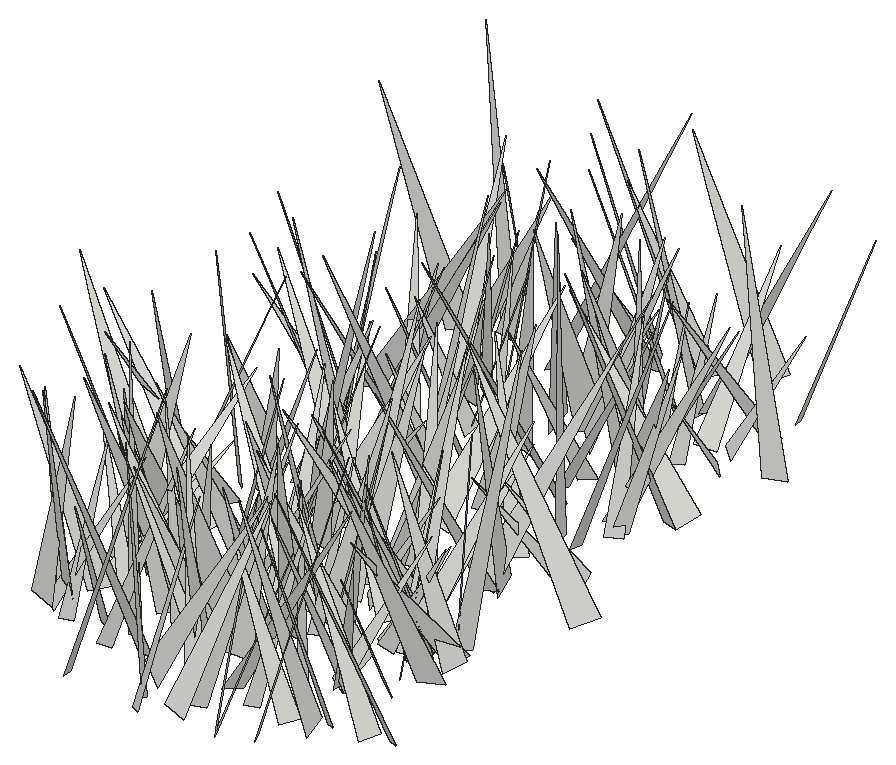
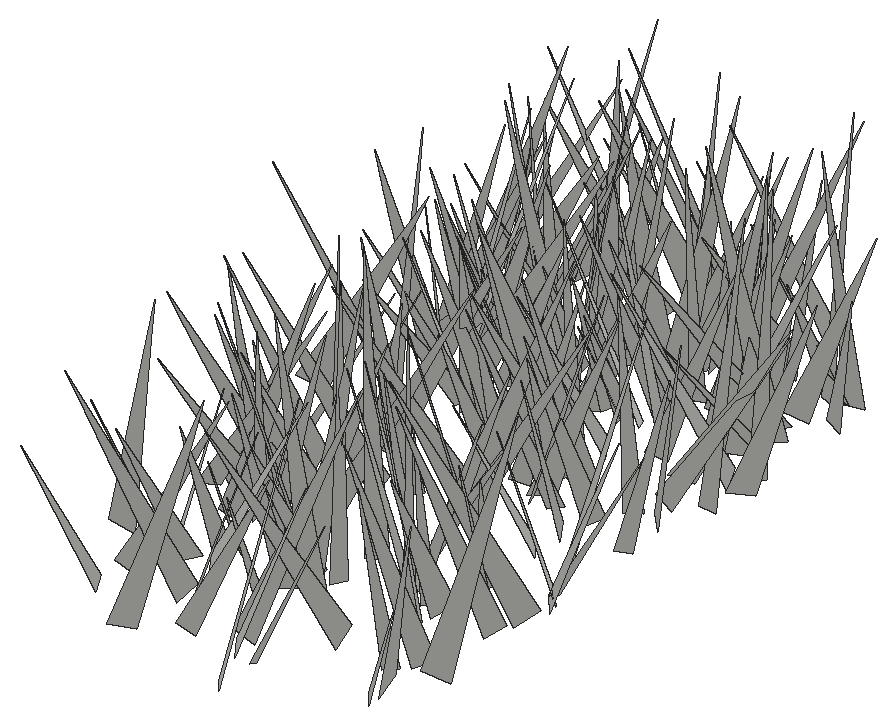
# SketchUp Ruby script. Lengths in inches.
U = 1.inch
M = Sketchup.active_model
def pt(a) = Geom::Point3d.new(a.map { |v| v * U })
def face(e, loops, mat)
  f = e.add_face(loops[0].map { |a| pt(a) })
  loops[1..].each { |l| e.add_face(l.map { |a| pt(a) }).erase! }
  f.material = f.back_material = mat if mat
  f
end
# faces: each face lists its corners as indices into pts; further lists are holes
def faces(e, pts, list, mat = nil) = list.each { |f| face(e, (f[0].is_a?(Array) ? f : [f]).map { |l| l.map { |i| pts[i] } }, mat) }
# xy, xz, yz: faces in a plane at the given z, y or x. An outline is a flat list of corners, or four numbers for a rectangle; further outlines are holes
def ring(l) = l.size == 4 ? [[l[0], l[1]], [l[2], l[1]], [l[2], l[3]], [l[0], l[3]]] : l.each_slice(2).to_a
def flat(e, list, mat, &to3) = list.each { |f| face(e, (f[0].is_a?(Array) ? f : [f]).map { |l| ring(l).map { |u, v| to3.(u, v) } }, mat) }
def xy(e, z, list, mat = nil) = flat(e, list, mat) { |x, y| [x, y, z] }
def xz(e, y, list, mat = nil) = flat(e, list, mat) { |x, z| [x, y, z] }
def yz(e, x, list, mat = nil) = flat(e, list, mat) { |y, z| [x, y, z] }
def lines(e, pts, list) = list.each { |a, b| e.add_line(pt(pts[a]), pt(pts[b])) }
# prism: a flat outline (further loops are holes) pulled along v
def prism(e, loops, v, mat = nil)
  f = face(e, loops, mat); d = Geom::Vector3d.new(v.map { |x| x * U })
  f.pushpull(f.normal.samedirection?(d) ? d.length : -d.length)
end
def box(e, o, s, mat = nil) = prism(e, [[o, [o[0] + s[0], o[1], o[2]], [o[0] + s[0], o[1] + s[1], o[2]], [o[0], o[1] + s[1], o[2]]]], [0, 0, s[2]], mat)
def at(x, y, z, deg = 0) = Geom::Transformation.translation(pt([x, y, z])) * Geom::Transformation.rotation(ORIGIN, Z_AXIS, deg.degrees)
def axes(o, x, y, z) = Geom::Transformation.new([*x, 0, *y, 0, *z, 0, *pt(o).to_a, 1])
def part(name) = M.definitions.add(name)
# library, detail: a bought-in or finely detailed component or shape, given as its bounding box
def library(name, o, s) = part(name).tap { |d| box(d.entities, o, s) }
def detail(e, o, s) = box(e.add_group.entities, o, s)
def put(e, d, t, mat = nil) = e.add_instance(d, t).tap { |i| i.material = mat if mat }
def group(e, t, mat = nil) = e.add_group.tap { |g| g.transformation = t; g.material = mat if mat }.entities
root = M.entities
c1 = part("fur_instance\#9")
p = [[0.8125,0,1.79],[0.67,-0.02,1.48],[0,-0.11,0],[0,0.11,0]]
faces(c1.entities,p,[[0,1,2,3]])
put(root,c1,axes([454.45,326.67,-21.66],[-5.80896,4.38047,0.69826],[4.41604,5.60261,1.59041],[-0.41794,-1.68592,7.09952]))
put(root,c1,axes([454.91,341.82,-21.66],[-4.61833,-3.74237,0.73758],[-3.79853,4.40694,-1.4242],[-0.34716,1.56584,5.77113]))
put(root,c1,axes([456,353.72,-21.66],[-7.80069,-0.47128,0.71432],[-0.70737,7.23754,-2.94972],[0.48165,2.99651,7.23686]))
put(root,c1,axes([454.72,351.37,-21.66],[1.74253,-7.39949,2.19817],[-7.33714,-2.28781,-1.88496],[-2.39807,1.62304,7.36449]))
put(root,c1,axes([455.25,340.96,-21.66],[-4.70731,-0.314,0.0439],[-0.28456,4.4722,1.47573],[0.13983,-1.46975,4.48103]))
put(root,c1,axes([455.15,318.15,-21.66],[0.45308,4.94253,1.25959],[4.74966,-0.86975,1.70432],[-1.859,-1.01755,4.66145]))
put(root,c1,axes([457.82,327.3125,-21.66],[-5.05806,4.73106,0.08976],[4.36112,4.60989,2.7757],[-1.83619,-2.08349,6.34527]))
put(root,c1,axes([456.97,329.83,-21.66],[-0.73144,-5.99959,0.26703],[-5.39662,0.53861,-2.681],[-2.63493,0.56233,5.41685]))
put(root,c1,axes([455.95,355.36,-21.66],[-3.1769,-1.92196,0.83625],[-2.09296,2.82701,-1.45378],[-0.11299,1.67333,3.4166]))
put(root,c1,axes([456.02,331.62,-21.66],[-4.69579,-3.74143,2.09942],[-4.25802,4.44495,-1.60248],[0.52452,2.58851,5.78625]))
put(root,c1,axes([457.25,318.62,-21.66],[-3.27496,5.22829,1.96451],[5.47571,2.5569,2.32348],[-1.10043,-2.83671,5.71505]))
put(root,c1,axes([455.21,341.04,-21.66],[4.3588,4.87451,1.02077],[4.50794,-4.43827,1.9448],[-2.11691,0.58556,6.24322]))
put(root,c1,axes([455.375,335.16,-21.66],[3.46395,-3.11936,0.86631],[-2.7787,-3.51575,-1.54862],[-1.66124,-0.62369,4.39672]))
put(root,c1,axes([454.77,328.99,-21.66],[-2.27672,-7.40144,1.23154],[-7.29478,2.48469,1.44709],[1.75622,0.72557,7.60728]))
put(root,c1,axes([456.03,339.17,-21.66],[-4.76858,-5.56642,0.65425],[-5.40433,4.79429,1.40014],[1.48534,-0.42682,7.19472]))
put(root,c1,axes([459.25,321.66,-21.66],[-5.59942,-5.49473,0.70955],[-5.42162,5.22657,-2.3104],[-1.14084,2.13071,7.49717]))
put(root,c1,axes([458.1,321.33,-21.66],[-3.16034,-1.96863,0.75138],[-2.10046,2.8354,-1.40585],[-0.16774,1.5852,3.44773]))
put(root,c1,axes([454.72,324.94,-21.66],[-1.50636,-7.45489,0.25307],[-6.77182,1.47502,3.14252],[3.12761,-0.39686,6.92598]))
put(root,c1,axes([458.41,342.57,-21.66],[-4.8792,2.06982,0.10093],[1.96371,4.70056,-1.46614],[0.66196,1.31208,5.09325]))
put(root,c1,axes([455.55,315.87,-21.66],[-0.42435,-6.57592,2.54627],[-6.78158,1.0798,1.65847],[1.93298,2.34469,6.37748]))
put(root,c1,axes([455.8,345.44,-21.66],[1.53162,3.70831,1.75315],[4.01532,-0.97314,-1.44953],[0.83802,-2.1148,3.74116]))
put(root,c1,axes([457.88,314.98,-21.66],[-4.70225,1.57903,0.9136],[0.9953,4.33742,-2.37389],[1.52885,2.03289,4.35536]))
put(root,c1,axes([459.29,318.37,-21.66],[-1.35626,4.67986,0.4324],[4.48876,1.15652,1.56235],[-1.3925,-0.82998,4.61514]))
put(root,c1,axes([455.82,325.75,-21.66],[6.85876,3.23862,0.41321],[3.02392,-6.66397,2.03701],[-1.23097,1.67477,7.30628]))
put(root,c1,axes([458.6875,345.74,-21.66],[-5.84983,3.65343,0.11485],[3.32744,5.4123,-2.68634],[1.51292,2.22277,6.35229]))
put(root,c1,axes([457.08,316.24,-21.66],[-3.46246,-6.72611,1.90114],[-6.59046,3.84836,1.61233],[2.32826,0.89059,7.39118]))
put(root,c1,axes([457.16,323.55,-21.66],[4.65411,-4.15615,0.09318],[-4.0063,-4.52139,-1.56511],[-1.10988,-1.10744,6.04026]))
put(root,c1,axes([456.25,322.54,-21.66],[-0.23722,4.19444,0.05409],[3.55446,0.22976,-2.22834],[2.22756,0.08005,3.56147]))
put(root,c1,axes([455.27,345.79,-21.66],[6.30652,-2.10429,0.15189],[-2.07978,-6.12031,1.56194],[0.35446,1.52876,6.46224]))
put(root,c1,axes([454.82,343.72,-21.66],[6.90826,-2.9112,0.5406],[-2.88435,-6.30625,2.89882],[0.66922,2.87186,6.91346]))
put(root,c1,axes([457.01,352.21,-21.66],[1.41484,-4.55258,1.06253],[-4.54528,-1.07998,1.42506],[1.09333,1.40157,4.54939]))
put(root,c1,axes([461.44,318.69,-21.66],[0.20171,6.63601,2.13173],[6.14884,-1.17367,3.07178],[-3.28217,-1.79094,5.8857]))
put(root,c1,axes([456.18,315.875,-21.66],[3.26284,4.45559,0.15103],[4.26787,-3.06768,-1.7017],[1.28856,-1.1217,5.25381]))
put(root,c1,axes([456,350.75,-21.66],[4.35594,-4.3452,0.48537],[-4.22774,-4.01128,2.03138],[1.11472,1.7662,5.80763]))
put(root,c1,axes([459.2,335.46,-21.66],[4.53649,3.63122,1.57008],[3.09166,-4.74451,2.04009],[-2.46831,0.73111,5.44092]))
put(root,c1,axes([456.54,321.33,-21.66],[0.11593,7.32982,3.76994],[7.80213,1.11829,-2.4142],[2.6581,-3.60212,6.9218]))
put(root,c1,axes([460.31,326.29,-21.66],[2.04194,-5.37013,1.21962],[-4.97283,-2.35693,-2.05211],[-2.36574,0.31918,5.36625]))
put(root,c1,axes([457.5,331.64,-21.66],[0.9975,-5.62203,0.93729],[-5.55991,-0.75041,1.41599],[1.25425,1.14473,5.53148]))
put(root,c1,axes([457.11,320.0625,-21.66],[-1.44675,6.62808,0.1342],[5.91861,1.35324,-3.03008],[2.98656,0.529,6.06986]))
put(root,c1,axes([462.35,333.15,-21.66],[-5.71185,4.45959,0.23835],[4.39877,5.55102,1.55146],[-0.77178,-1.36683,7.07857]))
put(root,c1,axes([458.05,324.46,-21.66],[7.18044,-3.7228,0.21814],[-3.29243,-6.55088,-3.42221],[-1.75122,-2.94828,7.32847]))
put(root,c1,axes([460.53,320.83,-21.66],[0.98136,-7.62341,0.77855],[-7.49654,-1.11781,-1.49599],[-1.58884,0.56543,7.53933]))
put(root,c1,axes([462.77,333.13,-21.66],[-7.75285,-2.01113,0.68817],[-2.11722,7.53738,-1.82488],[0.1887,1.94117,7.79879]))
put(root,c1,axes([461.73,315.84,-21.66],[2.76553,6.92914,2.18566],[6.51494,-3.40021,2.53621],[-3.21647,-0.92942,7.01632]))
put(root,c1,axes([459.09,337.72,-21.66],[4.51704,3.2359,0.24642],[3.07452,-4.40221,1.45028],[-1.0388,1.04161,5.3639]))
put(root,c1,axes([458.46,333.63,-21.66],[4.54931,-2.96003,1.24819],[-3.21199,-4.22741,1.68171],[-0.05363,2.09362,5.16041]))
put(root,c1,axes([463.15,340.97,-21.66],[-3.16767,-3.69393,0.44061],[-3.42422,2.66901,-2.24153],[-1.45395,1.76199,4.31912]))
put(root,c1,axes([463.41,314.64,-21.66],[-3.74944,-6.99723,1.04952],[-6.92154,3.38084,-2.18706],[-1.468,1.93125,7.63127]))
put(root,c1,axes([460.03,315.61,-21.66],[-1.799,-4.93024,0.4482],[-4.7112,1.85147,1.45641],[1.52075,-0.09654,5.04207]))
put(root,c1,axes([463.7,337.92,-21.66],[-2.5504,-6.61055,0.06946],[-6.29815,2.40698,-2.17909],[-2.00934,0.84606,6.74207]))
put(root,c1,axes([461.82,343.42,-21.66],[-4.35378,0.44066,1.23045],[0.84047,4.2213,1.46212],[1.0009,-1.62788,4.12453]))
put(root,c1,axes([460.77,331.1,-21.66],[7.1916,2.06862,2.54607],[1.20326,-7.37063,2.58975],[-3.05186,1.96861,7.0208]))
put(root,c1,axes([458.76,347.55,-21.66],[5.69332,3.04756,1.30745],[3.31373,-5.12843,-2.47574],[0.12746,-2.79687,5.96424]))
put(root,c1,axes([459.66,345.77,-21.66],[0.42063,-4.67833,0.35233],[-4.37367,-0.26302,1.72907],[1.69763,0.48155,4.36738]))
put(root,c1,axes([461.125,314.07,-21.66],[-5.44791,2.04028,1.98238],[0.64646,5.0587,-3.42987],[2.77031,2.83181,4.69878]))
put(root,c1,axes([462.67,331.28,-21.66],[-4.26385,3.34064,0.29483],[3.15748,4.15963,-1.468],[1.13011,0.98225,5.21395]))
put(root,c1,axes([463.83,316.89,-21.66],[-6.21207,0.31771,0.7174],[0.09871,5.99609,-1.80072],[0.77837,1.77522,5.95384]))
put(root,c1,axes([462.92,356.15,-21.66],[-3.99864,-1.03805,0.42764],[-0.78188,3.71014,1.695],[0.80565,-1.55139,3.76744]))
put(root,c1,axes([464.61,355.43,-21.66],[-5.23852,-3.39609,0.6769],[-3.443,4.97658,-1.67721],[-0.37061,1.77027,6.01352]))
put(root,c1,axes([461.47,310.59,-21.66],[6.96857,3.90701,1.2479],[3.36407,-6.85211,2.66731],[-2.34628,1.77954,7.53068]))
put(root,c1,axes([464.39,318.08,-21.66],[-6.62778,2.24684,1.33683],[2.5489,6.36376,1.94128],[0.58185,-2.2841,6.72363]))
put(root,c1,axes([460.31,346.55,-21.66],[-2.5118,-6.70095,1.69222],[-6.07027,2.9998,2.86854],[3.30427,0.41708,6.55616]))
put(root,c1,axes([464.28,337.13,-21.66],[-0.7633,-7.78268,1.04828],[-7.63293,0.4877,-1.93706],[-1.84592,1.20152,7.57632]))
put(root,c1,axes([462.84,359.08,-21.66],[-6.10663,-5.12788,1.30944],[-4.81653,6.21333,1.86984],[2.19336,-0.63253,7.75176]))
put(root,c1,axes([462.75,338.36,-21.66],[4.10406,6.33899,0.98584],[6.11766,-4.2195,1.66374],[-1.93105,0.10466,7.36601]))
put(root,c1,axes([461.02,351.08,-21.66],[7.74445,1.42991,0.81828],[1.0012,-7.20795,3.11989],[-1.30836,2.94814,7.231]))
put(root,c1,axes([463.49,343.16,-21.66],[5.66789,4.81372,1.80284],[4.22946,-5.89252,2.43659],[-2.92126,0.80836,7.02566]))
put(root,c1,axes([460.75,325.09,-21.66],[6.83601,2.20523,1.02382],[2.40175,-6.59991,-1.82073],[-0.37792,-2.05437,6.94831]))
put(root,c1,axes([462.76,327.26,-21.66],[5.4592,3.52611,0.65952],[3.05756,-5.20187,2.50265],[-1.87611,1.78282,5.99776]))
put(root,c1,axes([462.05,323.25,-21.66],[6.79493,0.95964,1.40947],[0.56386,-6.72962,1.86359],[-1.60922,1.6941,6.60447]))
put(root,c1,axes([460.98,333.67,-21.66],[0.71966,5.69009,1.64056],[5.43341,0.02279,-2.46251],[2.35511,-1.79132,5.17987]))
put(root,c1,axes([461.04,344.66,-21.66],[5.75664,2.23558,0.62086],[2.31995,-5.52205,-1.62697],[0.03364,-1.74108,5.95732]))
put(root,c1,axes([465.04,354.21,-21.66],[-0.88458,-7.33954,0.10795],[-7.20369,0.84713,-1.43254],[-1.40973,0.27658,7.25253]))
put(root,c1,axes([464.45,338.03,-21.66],[1.33499,-4.14938,1.03511],[-3.92508,-1.61935,-1.42916],[-1.69781,0.48101,4.1179]))
put(root,c1,axes([462.26,320.4,-21.66],[-0.76172,-5.93829,1.58025],[-5.83151,1.20063,1.7008],[1.93753,1.27903,5.74028]))
put(root,c1,axes([466.95,323.11,-21.66],[-5.54363,5.04114,0.10568],[4.92423,5.3789,1.72499],[-1.08457,-1.34553,7.29173]))
put(root,c1,axes([465.28,318.05,-21.66],[1.50286,-5.49819,1.33251],[-5.18917,-1.88889,-1.94134],[-2.25347,0.68284,5.35909]))
put(root,c1,axes([466.13,311.1,-21.66],[-6.09623,-2.24198,1.5344],[-2.70516,5.35755,-2.91953],[0.25098,3.28863,5.80232]))
put(root,c1,axes([464.22,324.01,-21.66],[-4.08665,1.67614,0.95166],[1.15635,3.91687,-1.93308],[1.54207,1.50482,3.97156]))
put(root,c1,axes([463.8,320.8,-21.66],[5.79186,-5.56058,1.06137],[-5.14067,-5.80215,-2.34538],[-2.37068,-1.00358,7.67886]))
put(root,c1,axes([464.09,332.76,-21.66],[4.06405,-3.6671,0.18626],[-3.28339,-3.75381,-2.26428],[-1.64366,-1.56845,4.98369]))
put(root,c1,axes([464.62,324.06,-21.66],[2.09645,3.63188,0.13416],[3.39461,-2.01213,1.42535],[-1.29816,0.60366,3.94386]))
put(root,c1,axes([465.27,323.62,-21.66],[-4.827,3.94667,0.05385],[3.76525,4.62978,-1.80751],[1.18405,1.36675,5.96733]))
put(root,c1,axes([462.75,321.3,-21.66],[4.25693,-2.37845,0.80532],[-2.50825,-3.95225,1.586],[0.11926,1.77474,4.61119]))
put(root,c1,axes([463.29,329.15,-21.66],[0.26156,-6.27199,1.2943],[-6.21893,0.06053,1.55008],[1.52905,1.31908,6.08306]))
put(root,c1,axes([466.35,339.27,-21.66],[1.43264,6.02249,0.66756],[5.77311,-1.565,1.72927],[-1.84042,-0.22107,5.94411]))
put(root,c1,axes([467.85,355.51,-21.66],[-2.55985,4.83206,1.74885],[4.89019,1.69025,2.4878],[-1.579,-2.59892,4.86955]))
put(root,c1,axes([462.39,330.15,-21.66],[3.74419,-3.98525,0.35569],[-3.51637,-3.04515,2.89653],[1.90889,2.20738,4.63803]))
put(root,c1,axes([467.35,313.7,-21.66],[0.02975,6.47261,1.15989],[6.34372,-0.33363,1.69906],[-1.73125,-1.11127,6.2457]))
put(root,c1,axes([465.97,324.68,-21.66],[6.61822,-2.56323,1.80089],[-1.74555,-6.51281,-2.85492],[-2.60123,-2.15113,6.49773]))
put(root,c1,axes([462.99,324.16,-21.66],[5.8637,3.4963,0.04079],[3.31459,-5.53283,-2.23832],[1.11324,-1.94227,6.44958]))
put(root,c1,axes([464.78,346.78,-21.66],[7.73874,0.04549,1.82687],[0.5794,-7.60007,-2.26513],[-1.73315,-2.33761,7.39995]))
put(root,c1,axes([465.82,348.07,-21.66],[6.63906,-4.24471,1.17982],[-3.75911,-6.57064,-2.48644],[-2.29753,-1.51516,7.47745]))
put(root,c1,axes([466.73,331.93,-21.66],[-5.00496,1.9066,1.35129],[1.19771,4.83542,-2.3864],[2.00664,1.8693,4.79477]))
put(root,c1,axes([466.52,309.85,-21.66],[3.68113,4.53912,0.36663],[4.24955,-3.59341,1.82137],[-1.63686,0.87892,5.5531]))
put(root,c1,axes([469.94,340.55,-21.66],[-3.80092,-6.72254,0.0507],[-6.48684,3.65215,-2.05545],[-1.76524,1.05421,7.4441]))
put(root,c1,axes([464.75,343.61,-21.66],[-0.13317,-8.12567,1.45261],[-7.87911,0.55826,2.40046],[2.46092,1.34765,7.76415]))
put(root,c1,axes([469.95,351.98,-21.66],[-6.83624,-2.0461,0.45627],[-2.08301,6.45462,-2.26447],[-0.23611,2.29788,6.76704]))
put(root,c1,axes([466.48,315.76,-21.66],[6.75782,0.35235,2.65885],[1.16075,-6.88187,-2.03823],[-2.41791,-2.31896,6.45275]))
put(root,c1,axes([467.33,350.28,-21.66],[3.33394,1.47543,1.26624],[0.9738,-3.44268,1.44745],[-1.68284,0.93087,3.34618]))
put(root,c1,axes([465.17,348.33,-21.66],[0.9927,-7.18833,2.00129],[-7.23058,-0.4281,2.04891],[1.84279,2.19257,6.96128]))
put(root,c1,axes([467.72,324.23,-21.66],[-6.44031,-4.10602,1.97316],[-3.85542,6.73281,1.42663],[2.42663,-0.20036,7.50344]))
put(root,c1,axes([471.05,349.5,-21.66],[-6.43148,-3.95381,0.27263],[-3.76371,5.93049,-2.78112],[-1.24153,2.50351,7.01869]))
put(root,c1,axes([467.82,325.64,-21.66],[-7.05102,3.6652,1.50452],[2.87345,6.84526,-3.20935],[2.72774,2.26338,7.26985]))
put(root,c1,axes([467.38,331.29,-21.66],[5.51307,6.12337,0.96272],[5.81555,-5.55551,2.03274],[-2.14519,0.67601,7.98483]))
put(root,c1,axes([466.52,348.85,-21.66],[-0.20342,5.45726,1.92359],[5.57072,0.70526,-1.41173],[1.56492,-1.80117,5.27542]))
put(root,c1,axes([467.47,324.01,-21.66],[-4.01189,-2.17426,1.82805],[-1.57492,4.33524,1.69992],[2.36407,-0.80168,4.23473]))
put(root,c1,axes([467.43,319.64,-21.66],[6.21031,-0.46369,2.15458],[0.49806,-5.98034,-2.72263],[-2.14689,-2.7287,5.60092]))
put(root,c1,axes([466.07,346.81,-21.66],[4.34648,-1.55951,0.20323],[-1.53377,-4.07129,1.56122],[0.34774,1.53551,4.34586]))
put(root,c1,axes([466.51,334.57,-21.66],[-0.73588,7.38124,0.25307],[6.98236,0.77818,-2.39362],[2.40696,-0.00075,7.02103]))
put(root,c1,axes([467.32,327.34,-21.66],[5.50822,-3.47682,2.75588],[-4.25576,-5.38219,1.71589],[-1.25366,2.99458,6.28367]))
put(root,c1,axes([470.95,325.27,-21.66],[-3.6214,4.75768,0.36392],[4.63089,3.39426,1.70771],[-1.15013,-1.31374,5.73008]))
put(root,c1,axes([470.51,344.94,-21.66],[-3.32037,-5.8988,2.51801],[-6.36421,2.67847,-2.11746],[-0.7956,3.19234,6.42939]))
put(root,c1,axes([468.86,321.72,-21.66],[-4.41847,1.33903,1.10997],[0.76139,4.21375,-2.05244],[1.56375,1.73183,4.13562]))
put(root,c1,axes([470.64,357.3,-21.66],[-5.74656,4.30747,2.03787],[4.75581,5.38477,2.02895],[0.29923,-2.86007,6.88916]))
put(root,c1,axes([469.65,343.16,-21.66],[1.26749,-5.25605,0.55346],[-5.00773,-1.37633,-1.60227],[-1.68968,0.13629,5.16385]))
put(root,c1,axes([467.13,317.45,-21.66],[2.95876,-6.29379,1.88961],[-6.54545,-2.63888,1.45948],[0.58268,2.31543,6.79971]))
put(root,c1,axes([464.87,313.26,-21.66],[4.40787,6.56573,1.54887],[6.23945,-3.26461,-3.91775],[2.5646,-3.34225,6.86945]))
put(root,c1,axes([467.67,329.66,-21.66],[6.41211,-0.61612,1.30158],[-0.93497,-6.2989,1.62436],[-1.09524,1.77006,6.23347]))
put(root,c1,axes([470.96,328.05,-21.66],[-6.61706,2.95045,0.41304],[2.75432,6.44194,-1.89112],[1.13554,1.56763,6.99387]))
put(root,c1,axes([468.71,312,-21.66],[7.42059,-0.17453,3.00871],[-1.57677,-7.03899,3.48057],[-2.56838,3.81708,6.55601]))
put(root,c1,axes([467.47,330.375,-21.66],[2.98572,-5.88102,1.99527],[-6.13329,-2.44486,1.97166],[0.97482,2.63026,6.29392]))
put(root,c1,axes([468.05,320.89,-21.66],[0.34985,-8.1007,0.677],[-7.9597,-0.20383,1.67442],[1.6501,0.73429,7.93347]))
put(root,c1,axes([467.65,337.29,-21.66],[4.01839,-5.64573,1.18023],[-5.73753,-3.76564,1.52164],[0.58986,1.83314,6.76065]))
put(root,c1,axes([472.6,326.47,-21.66],[1.75618,-7.20882,1.45322],[-6.25973,-2.24953,-3.59425],[-3.85938,0.3683,6.49097]))
put(root,c1,axes([468.27,310.9,-21.66],[1.11802,6.55656,0.88639],[6.4324,-0.86675,-1.70208],[1.54866,-1.13332,6.42972]))
put(root,c1,axes([467.18,346.18,-21.66],[5.13352,5.29295,1.04527],[5.31008,-4.70157,-2.27141],[0.95446,-2.31104,7.01492]))
put(root,c1,axes([471.95,334.54,-21.66],[-1.56415,5.71782,0.81541],[5.62888,1.31989,1.54221],[-1.29382,-1.17019,5.72377]))
put(root,c1,axes([471.47,317.4,-21.66],[-5.20455,-0.25594,1.25726],[-0.61037,5.11409,-1.48563],[1.12857,1.58561,4.99457]))
put(root,c1,axes([471.03,347.2,-21.66],[1.74005,3.73475,0.21366],[3.48509,-1.70407,1.40429],[-1.35946,0.41179,3.87351]))
put(root,c1,axes([473.01,330.94,-21.66],[-1.63485,-6.2778,0.46595],[-5.97391,1.39539,-2.16005],[-1.98499,0.97094,6.117]))
put(root,c1,axes([472.77,320.95,-21.66],[-6.88482,-1.0416,0.48285],[-0.90858,6.73783,1.57954],[0.70182,-1.49517,6.78165]))
put(root,c1,axes([471.2,310.63,-21.66],[4.43621,4.25023,1.48293],[3.65379,-4.61591,2.29927],[-2.62932,0.75659,5.69717]))
put(root,c1,axes([471.03,313.84,-21.66],[-4.89219,1.92037,1.37183],[1.09822,4.64707,-2.5888],[2.08893,2.05431,4.57377]))
put(root,c1,axes([468.78,322.96,-21.66],[1.45839,-7.20301,2.88114],[-7.56056,-0.66269,2.17028],[1.73849,3.16049,7.02141]))
put(root,c1,axes([469.2,341.57,-21.66],[5.44463,0.12063,0.24069],[0.04962,-5.23956,1.50366],[-0.26462,1.49964,5.23426]))
put(root,c1,axes([472.52,337.35,-21.66],[-7.45834,-2.27512,2.73301],[-2.96816,7.48025,-1.87304],[1.95846,2.67246,7.56933]))
put(root,c1,axes([468.86,326.14,-21.66],[3.3459,3.39415,0.39754],[3.18536,-2.89609,-2.08314],[1.23764,-1.72213,4.2867]))
put(root,c1,axes([472.45,343.61,-21.66],[-6.55431,0.09701,1.7896],[-0.34688,6.588,-1.62754],[1.75834,1.66126,6.34976]))
put(root,c1,axes([468.66,323.75,-21.66],[7.66511,2.45698,1.17946],[2.70747,-7.26796,-2.45522],[-0.3122,-2.70587,7.66567]))
put(root,c1,axes([473.59,313.74,-21.66],[-3.5373,3.73043,1.14853],[3.88761,3.22863,1.48666],[-0.34887,-1.84596,4.92122]))
put(root,c1,axes([473.46,344.78,-21.66],[-0.04463,-6.97717,1.39975],[-6.92736,-0.27772,-1.60522],[-1.62845,1.37265,6.79015]))
put(root,c1,axes([472.21,347.26,-21.66],[-4.0426,1.99311,1.15136],[1.52694,4.06338,-1.67276],[1.72237,1.07573,4.18533]))
put(root,c1,axes([469.09,314.6875,-21.66],[6.564,-1.73993,0.0582],[-1.67851,-6.26496,2.01239],[0.46191,1.95953,6.48565]))
put(root,c1,axes([471.41,310.33,-21.66],[4.34106,2.99141,0.28027],[2.79242,-4.19877,1.56351],[-1.10882,1.13738,5.03476]))
put(root,c1,axes([469.33,337.63,-21.66],[7.73901,0.54751,0.09462],[0.50511,-7.48314,1.98706],[-0.23147,1.9758,7.49957]))
put(root,c1,axes([472.83,325.11,-21.66],[2.63198,-5.20128,0.6124],[-4.94839,-2.69423,-1.6156],[-1.71515,-0.20845,5.60093]))
put(root,c1,axes([474.2,317.96,-21.66],[-1.75901,-5.06572,0.78099],[-4.97011,1.48393,-1.5689],[-1.25276,1.22556,5.12778]))
put(root,c1,axes([470.58,322.36,-21.66],[4.65665,4.64477,2.8893],[5.46904,-4.02795,-2.33914],[-0.10763,-3.71592,6.14709]))
put(root,c1,axes([470.14,352.54,-21.66],[7.35163,-0.33714,0.71191],[-0.54127,-7.01692,2.26646],[-0.57229,2.30568,7.00167]))
put(root,c1,axes([472.29,349.51,-21.66],[-2.9389,4.8588,0.20427],[4.55933,2.83593,-1.85926],[1.6918,0.79774,5.36547]))
put(root,c1,axes([474.47,352.36,-21.66],[0.43766,-5.35462,0.13989],[-4.92597,-0.45748,-2.09965],[-2.10387,-0.04276,4.94519]))
put(root,c1,axes([475.43,314.77,-21.66],[-3.98273,-4.40716,0.90523],[-4.3967,3.55588,-2.0321],[-0.95477,2.0093,5.58174]))
put(root,c1,axes([471.61,327.96,-21.66],[-2.11402,4.56513,0.60738],[3.84978,2.11854,-2.52378],[2.52756,0.59144,4.35202]))
put(root,c1,axes([473.9375,323.01,-21.66],[1.42623,8.08681,0.06748],[7.92603,-1.41139,1.61901],[-1.60595,0.21606,8.05043]))
put(root,c1,axes([474.0625,324.92,-21.66],[-5.99255,-5.60768,0.41861],[-5.37957,5.89507,1.95969],[1.63755,-1.155,7.96972]))
put(root,c1,axes([476.5,342.87,-21.66],[-6.39943,2.86094,0.01202],[2.71801,6.07041,2.2137],[-0.89308,-2.0256,6.65111]))
put(root,c1,axes([475.91,342.02,-21.66],[-4.08084,-6.31933,0.93728],[-6.28934,3.77891,-1.90517],[-1.12095,1.80323,7.27719]))
put(root,c1,axes([471.79,327.55,-21.66],[1.01067,5.88602,0.15693],[5.68933,-0.93518,-1.56469],[1.51703,-0.41415,5.76354]))
put(root,c1,axes([474.54,339.18,-21.66],[-5.37291,2.30629,0.61766],[1.96946,5.14098,-2.06404],[1.34972,1.6793,5.47055]))
put(root,c1,axes([474.51,334.55,-21.66],[-4.21387,-1.59887,0.24339],[-1.27519,3.70248,2.24451],[0.99474,-2.02671,3.90836]))
put(root,c1,axes([473.72,323.1,-21.66],[-3.75985,-4.2409,1.14983],[-3.97997,3.92819,1.47409],[1.86202,-0.16705,5.47255]))
put(root,c1,axes([473.3125,331.7,-21.66],[-6.68782,-2.79113,3.18251],[-2.04813,7.34131,2.13449],[3.70459,-0.98003,6.92541]))
put(root,c1,axes([474.93,314.08,-21.66],[-7.14717,-1.7401,1.8273],[-1.33254,7.26397,1.70532],[2.14274,-1.28679,7.15555]))
put(root,c1,axes([473.24,311.46,-21.66],[6.6915,4.26773,1.20587],[3.94044,-6.72308,1.92792],[-2.03484,1.01512,7.69888]))
put(root,c1,axes([477.8,315.02,-21.66],[-2.08516,6.03207,0.25096],[5.29839,1.7011,3.1353],[-2.89412,-1.23172,5.5591]))
put(root,c1,axes([472.51,342.77,-21.66],[5.53562,0.75174,0.06867],[0.66774,-5.11345,2.14935],[-0.35205,2.12143,5.1564]))
put(root,c1,axes([472.33,323.1,-21.66],[1.50617,-3.93782,1.16858],[-3.70084,-0.76096,2.20573],[1.78207,1.74788,3.59301]))
put(root,c1,axes([474.22,348.16,-21.66],[-2.58943,-3.13022,0.07236],[-2.65217,2.2427,2.10831],[1.66419,-1.2964,3.47253]))
put(root,c1,axes([472.62,322.86,-21.66],[1.91277,-3.82749,0.78831],[-3.61325,-1.39793,1.9799],[1.48846,1.5251,3.7932]))
put(root,c1,axes([475.08,320.92,-21.66],[4.44395,3.96646,1.43413],[3.47391,-4.62357,2.02305],[-2.39195,0.65422,5.60257]))
put(root,c1,axes([473.61,337.24,-21.66],[6.82922,2.21825,1.16198],[1.82522,-6.72015,2.10172],[-1.71447,1.68168,6.86597]))
put(root,c1,axes([475.22,323.44,-21.66],[-4.26482,-5.03014,0.77761],[-4.82923,4.31941,1.45497],[1.60794,-0.36894,6.43227]))
put(root,c1,axes([473.22,318.57,-21.66],[5.22724,-1.35677,0.09683],[-1.28473,-5.05093,-1.4184],[-0.44684,-1.34966,5.21086]))
put(root,c1,axes([472,343.49,-21.66],[1.01842,-6.5564,0.3467],[-5.92672,-0.76709,2.90332],[2.82498,0.75429,5.9661]))
put(root,c1,axes([476.19,334.89,-21.66],[-4.14982,-0.72477,0.23143],[-0.53834,3.70403,1.94686],[0.53763,-1.88541,3.73578]))
put(root,c1,axes([478.96,331.28,-21.66],[-4.49913,6.58347,1.21187],[6.27218,3.63575,3.53468],[-2.33889,-2.91414,7.14775]))
put(root,c1,axes([473.07,318.32,-21.66],[2.06268,4.77096,0.10661],[4.57909,-1.94603,-1.50762],[1.34363,-0.69206,4.97431]))
put(root,c1,axes([474.39,354.51,-21.66],[4.68389,2.5085,0.46697],[2.25732,-4.52881,1.68637],[-1.1896,1.28326,5.03861]))
put(root,c1,axes([472.15,331.52,-21.66],[2.96543,7.80813,0.73471],[7.53088,-2.61577,-2.59693],[2.18919,-1.57838,7.9383]))
put(root,c1,axes([476.51,323.73,-21.66],[3.82585,4.29132,1.89582],[3.55577,-4.24822,2.44044],[-3.06039,0.42878,5.20545]))
put(root,c1,axes([476.65,323.46,-21.66],[-6.00437,2.1113,1.91932],[2.55574,5.96789,1.43049],[1.26869,-2.0299,6.20191]))
put(root,c1,axes([474.47,339.74,-21.66],[4.97283,-0.90694,1.68915],[-1.45035,-4.85051,1.66547],[-1.25389,2.01364,4.77261]))
put(root,c1,axes([475.8,325.12,-21.66],[7.23662,0.86237,3.59764],[-0.54989,-7.56504,2.91946],[-3.65846,2.84288,6.67751]))
put(root,c1,axes([476.71,321.43,-21.66],[0.82289,-7.98079,0.80674],[-7.83354,-0.97405,-1.64552],[-1.72608,0.61581,7.85254]))
put(root,c1,axes([479.12,315.3,-21.66],[-4.75874,-5.64309,0.42264],[-5.39038,4.3522,-2.58279],[-1.72245,1.97043,6.91515]))
put(root,c1,axes([476.39,324.12,-21.66],[3.78174,-4.82109,0.17581],[-4.12071,-3.34423,-3.06777],[-2.50869,-1.77444,5.30408]))
put(root,c1,axes([473.56,349.79,-21.66],[2.80072,3.68056,0.20092],[3.50306,-2.57922,-1.58339],[1.14693,-1.10998,4.34551]))
put(root,c1,axes([477.17,349.12,-21.66],[-0.80473,7.1427,2.6366],[7.51279,0.31449,1.44102],[-1.23607,-2.73867,7.04196]))
put(root,c1,axes([475.41,319.51,-21.66],[-2.3415,-4.6423,0.1365],[-4.37976,2.25803,1.66471],[1.54509,-0.63449,4.92568]))
put(root,c1,axes([473.63,340.39,-21.66],[5.89458,-2.32049,1.52507],[-2.76984,-5.16651,2.8446],[-0.1962,3.22166,5.6603]))
